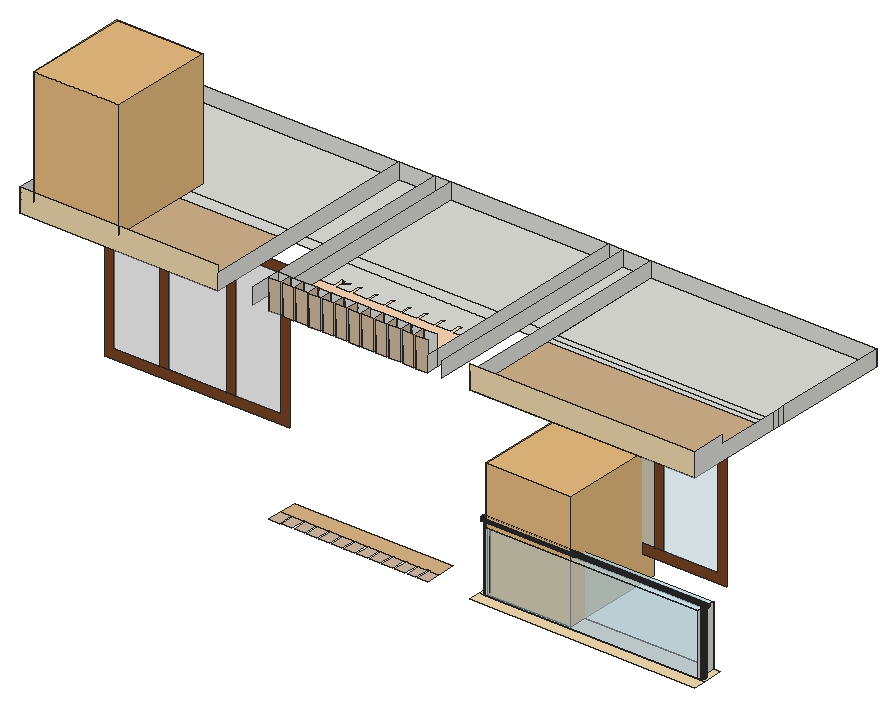
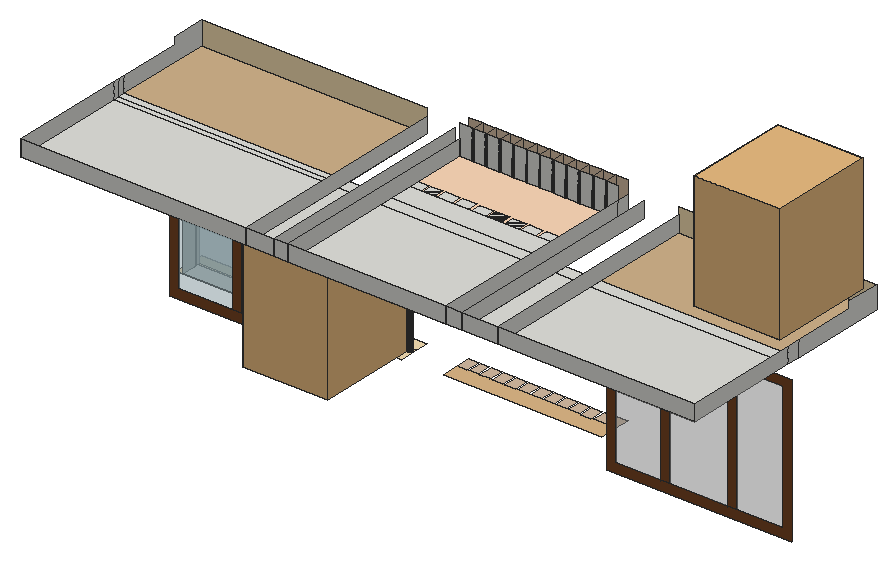
# SketchUp Ruby script. Lengths in inches.
U = 1.inch
M = Sketchup.active_model
def pt(a) = Geom::Point3d.new(a.map { |v| v * U })
def face(e, loops, mat)
  f = e.add_face(loops[0].map { |a| pt(a) })
  loops[1..].each { |l| e.add_face(l.map { |a| pt(a) }).erase! }
  f.material = f.back_material = mat if mat
  f
end
# faces: each face lists its corners as indices into pts; further lists are holes
def faces(e, pts, list, mat = nil) = list.each { |f| face(e, (f[0].is_a?(Array) ? f : [f]).map { |l| l.map { |i| pts[i] } }, mat) }
# xy, xz, yz: faces in a plane at the given z, y or x. An outline is a flat list of corners, or four numbers for a rectangle; further outlines are holes
def ring(l) = l.size == 4 ? [[l[0], l[1]], [l[2], l[1]], [l[2], l[3]], [l[0], l[3]]] : l.each_slice(2).to_a
def flat(e, list, mat, &to3) = list.each { |f| face(e, (f[0].is_a?(Array) ? f : [f]).map { |l| ring(l).map { |u, v| to3.(u, v) } }, mat) }
def xy(e, z, list, mat = nil) = flat(e, list, mat) { |x, y| [x, y, z] }
def xz(e, y, list, mat = nil) = flat(e, list, mat) { |x, z| [x, y, z] }
def yz(e, x, list, mat = nil) = flat(e, list, mat) { |y, z| [x, y, z] }
def lines(e, pts, list) = list.each { |a, b| e.add_line(pt(pts[a]), pt(pts[b])) }
# prism: a flat outline (further loops are holes) pulled along v
def prism(e, loops, v, mat = nil)
  f = face(e, loops, mat); d = Geom::Vector3d.new(v.map { |x| x * U })
  f.pushpull(f.normal.samedirection?(d) ? d.length : -d.length)
end
def box(e, o, s, mat = nil) = prism(e, [[o, [o[0] + s[0], o[1], o[2]], [o[0] + s[0], o[1] + s[1], o[2]], [o[0], o[1] + s[1], o[2]]]], [0, 0, s[2]], mat)
def at(x, y, z, deg = 0) = Geom::Transformation.translation(pt([x, y, z])) * Geom::Transformation.rotation(ORIGIN, Z_AXIS, deg.degrees)
def axes(o, x, y, z) = Geom::Transformation.new([*x, 0, *y, 0, *z, 0, *pt(o).to_a, 1])
def part(name) = M.definitions.add(name)
# library, detail: a bought-in or finely detailed component or shape, given as its bounding box
def library(name, o, s) = part(name).tap { |d| box(d.entities, o, s) }
def detail(e, o, s) = box(e.add_group.entities, o, s)
def put(e, d, t, mat = nil) = e.add_instance(d, t).tap { |i| i.material = mat if mat }
def group(e, t, mat = nil) = e.add_group.tap { |g| g.transformation = t; g.material = mat if mat }.entities
root = M.entities
M.materials.add("[0027_PeachPuff]").color = [255, 218, 185]
M.materials.add("[0034_Wheat]").color = [245, 222, 179]
M.materials.add("[0035_Tan]").color = [210, 180, 140]
M.materials.add("[0036_BurlyWood]1").color = [222, 184, 135]
M.materials.add("[Formica Laminate Dark]").color = [50, 53, 60]
M.materials.add("[Formica Laminate Light]").color = [213, 189, 164]
M.materials.add("[Translucent Glass Gray]").color = [191, 191, 191]
M.materials["[Translucent Glass Gray]"].alpha = 0.5
M.materials.add("[Translucent Glass Safety]").color = [204, 235, 244]
M.materials["[Translucent Glass Safety]"].alpha = 0.5
M.materials.add("[Wood Veneer 01]").color = [120, 70, 37]
c1 = library("chau cay",[-24.34,-109.24,0],[56.46,62.58,79.69])
xy(root,3893.0625,[[1416.35,332.76,2049.02,390.27],[1408.91,338.29,1408.19,338.33,1407.48,338.45,1406.79,338.64,1406.12,338.91,1405.48,339.24,1404.88,339.64,1404.33,340.1,1403.82,340.61,1403.375,341.18,1402.99,341.79,1402.67,342.43,1402.42,343.1,1402.24,343.8,1402.14,344.51,1402.11,345.23,1402.15,345.95,1402.27,346.66,1402.46,347.35,1402.73,348.02,1403.0625,348.66,1403.46,349.26,1403.92,349.8125,1404.43,350.32,1405,350.76,1405.6,351.15,1406.25,351.47,1406.92,351.72,1407.62,351.9,1408.33,352.01,1409.05,352.04,1409.77,351.99,1410.48,351.87,1411.17,351.68,1411.84,351.41,1412.47,351.07,1413.08,350.68,1413.63,350.22,1414.14,349.71,1414.58,349.14,1414.97,348.54,1415.29,347.89,1415.54,347.22,1415.72,346.52,1415.82,345.81,1415.85,345.09,1415.81,344.37,1415.6875,343.66,1415.5,342.97,1415.23,342.3,1414.9,341.66,1414.5,341.0625,1414.04,340.51,1413.53,340,1412.96,339.56,1412.36,339.17,1411.71,338.85,1411.04,338.6,1410.34,338.42,1409.63,338.32],[2056.54,338.29,2055.82,338.32,2055.11,338.4375,2054.42,338.62,2053.75,338.88,2053.1,339.21,2052.5,339.6,2051.94,340.05,2051.43,340.5625,2050.98,341.12,2050.59,341.72,2050.26,342.36,2050,343.04,2049.82,343.73,2049.7,344.44,2049.67,345.16,2049.7,345.88,2049.82,346.59,2050,347.29,2050.26,347.96,2050.59,348.6,2050.98,349.2,2051.43,349.76,2051.94,350.27,2052.5,350.72,2053.1,351.11,2053.75,351.44,2054.42,351.7,2055.11,351.89,2055.82,352,2056.54,352.04,2057.26,352,2057.97,351.89,2058.67,351.7,2059.34,351.44,2059.98,351.11,2060.58,350.72,2061.14,350.27,2061.65,349.76,2062.1,349.2,2062.5,348.6,2062.82,347.96,2063.08,347.29,2063.27,346.59,2063.38,345.88,2063.42,345.16,2063.38,344.44,2063.27,343.73,2063.08,343.04,2062.82,342.36,2062.5,341.72,2062.1,341.12,2061.65,340.5625,2061.14,340.05,2060.58,339.6,2059.98,339.21,2059.34,338.88,2058.67,338.62,2057.97,338.4375,2057.26,338.32]])
xy(root,3893.0625,[[1398.32,295.82,2069.85,332.76],[[1398.32,332.76,1416.35,390.27],[1408.91,338.29,1408.19,338.33,1407.48,338.45,1406.79,338.64,1406.12,338.91,1405.48,339.24,1404.88,339.64,1404.33,340.1,1403.82,340.61,1403.375,341.18,1402.99,341.79,1402.67,342.43,1402.42,343.1,1402.24,343.8,1402.14,344.51,1402.11,345.23,1402.15,345.95,1402.27,346.66,1402.46,347.35,1402.73,348.02,1403.0625,348.66,1403.46,349.26,1403.92,349.8125,1404.43,350.32,1405,350.76,1405.6,351.15,1406.25,351.47,1406.92,351.72,1407.62,351.9,1408.33,352.01,1409.05,352.04,1409.77,351.99,1410.48,351.87,1411.17,351.68,1411.84,351.41,1412.47,351.07,1413.08,350.68,1413.63,350.22,1414.14,349.71,1414.58,349.14,1414.97,348.54,1415.29,347.89,1415.54,347.22,1415.72,346.52,1415.82,345.81,1415.85,345.09,1415.81,344.37,1415.6875,343.66,1415.5,342.97,1415.23,342.3,1414.9,341.66,1414.5,341.0625,1414.04,340.51,1413.53,340,1412.96,339.56,1412.36,339.17,1411.71,338.85,1411.04,338.6,1410.34,338.42,1409.63,338.32]],[[2049.02,332.76,2069.85,390.27],[2056.54,338.29,2055.82,338.32,2055.11,338.4375,2054.42,338.62,2053.75,338.88,2053.1,339.21,2052.5,339.6,2051.94,340.05,2051.43,340.5625,2050.98,341.12,2050.59,341.72,2050.26,342.36,2050,343.04,2049.82,343.73,2049.7,344.44,2049.67,345.16,2049.7,345.88,2049.82,346.59,2050,347.29,2050.26,347.96,2050.59,348.6,2050.98,349.2,2051.43,349.76,2051.94,350.27,2052.5,350.72,2053.1,351.11,2053.75,351.44,2054.42,351.7,2055.11,351.89,2055.82,352,2056.54,352.04,2057.26,352,2057.97,351.89,2058.67,351.7,2059.34,351.44,2059.98,351.11,2060.58,350.72,2061.14,350.27,2061.65,349.76,2062.1,349.2,2062.5,348.6,2062.82,347.96,2063.08,347.29,2063.27,346.59,2063.38,345.88,2063.42,345.16,2063.38,344.44,2063.27,343.73,2063.08,343.04,2062.82,342.36,2062.5,341.72,2062.1,341.12,2061.65,340.5625,2061.14,340.05,2060.58,339.6,2059.98,339.21,2059.34,338.88,2058.67,338.62,2057.97,338.4375,2057.26,338.32]]],"[0034_Wheat]")
xy(root,3896.1875,[[800.41,338.63,1272.8,390.27]],"[0036_BurlyWood]1")
xy(root,3896.1875,[[800.41,295.82,831.22,338.63],[837.47,295.82,868.28,338.63],[875.6,295.82,906.41,338.63],[912.41,295.82,943.22,338.63],[949.16,295.82,979.97,338.63],
  [986.78,295.82,1017.6,338.63],[1024.35,295.82,1055.16,338.63],[1062.53,295.82,1093.35,338.63],[1100.28,295.82,1131.1,338.63],[1137.66,295.82,1168.47,338.63],
  [1175.22,295.82,1206.03,338.63],[1212.97,295.82,1238.19,338.63],[1243.78,295.82,1272.8,338.63]],"[Formica Laminate Light]")
xy(root,4072.9375,[[1416.35,332.76,2049.02,390.27]],"[Translucent Glass Safety]")
xy(root,4084.625,[[2056.54,338.29,2057.26,338.32,2057.97,338.4375,2058.67,338.62,2059.34,338.88,2059.98,339.21,2060.58,339.6,2061.14,340.05,2061.65,340.5625,2062.1,341.12,2062.5,341.72,2062.82,342.36,2063.08,343.04,2063.27,343.73,2063.38,344.44,2063.42,345.16,2063.38,345.88,2063.27,346.59,2063.08,347.29,2062.82,347.96,2062.5,348.6,2062.1,349.2,2061.65,349.76,2061.14,350.27,2060.58,350.72,2059.98,351.11,2059.34,351.44,2058.67,351.7,2057.97,351.89,2057.26,352,2056.54,352.04,2055.82,352,2055.11,351.89,2054.42,351.7,2053.75,351.44,2053.1,351.11,2052.5,350.72,2051.94,350.27,2051.43,349.76,2050.98,349.2,2050.59,348.6,2050.26,347.96,2050,347.29,2049.82,346.59,2049.7,345.88,2049.67,345.16,2049.7,344.44,2049.82,343.73,2050,343.04,2050.26,342.36,2050.59,341.72,2050.98,341.12,2051.43,340.5625,2051.94,340.05,2052.5,339.6,2053.1,339.21,2053.75,338.88,2054.42,338.62,2055.11,338.4375,2055.82,338.32]])
xy(root,4092.45,[[1408.91,338.29,1409.63,338.32,1410.34,338.42,1411.04,338.6,1411.71,338.85,1412.36,339.17,1412.96,339.56,1413.53,340,1414.04,340.51,1414.5,341.0625,1414.9,341.66,1415.23,342.3,1415.5,342.97,1415.6875,343.66,1415.81,344.37,1415.85,345.09,1415.82,345.81,1415.72,346.52,1415.54,347.22,1415.29,347.89,1414.97,348.54,1414.58,349.14,1414.42,349.34,1403.53,349.34,1403.46,349.26,1403.0625,348.66,1402.73,348.02,1402.46,347.35,1402.27,346.66,1402.15,345.95,1402.11,345.23,1402.14,344.51,1402.24,343.8,1402.42,343.1,1402.67,342.43,1402.99,341.79,1403.375,341.18,1403.82,340.61,1404.33,340.1,1404.88,339.64,1405.48,339.24,1406.12,338.91,1406.79,338.64,1407.48,338.45,1408.19,338.33],[1403.53,349.34,1414.42,349.34,1414.14,349.71,1413.63,350.22,1413.08,350.68,1412.47,351.07,1411.84,351.41,1411.17,351.68,1410.48,351.87,1409.77,351.99,1409.05,352.04,1408.33,352.01,1407.62,351.9,1406.92,351.72,1406.25,351.47,1405.6,351.15,1405,350.76,1404.43,350.32,1403.92,349.8125]])
xy(root,4453.25,[[800.41,483.92,800.41,584.29,1272.8,584.29,1272.8,483.92,1241.74,483.92,1241.74,514.17,1235.22,514.17,1235.22,483.92,1200.46,483.92,1200.46,514.17,1190.9375,514.17,1190.9375,483.92,1149.66,483.92,1149.66,514.17,1140.875,514.17,1140.875,483.92,1099.6,483.92,1099.6,514.17,1090.625,514.17,1090.625,483.92,1049.35,483.92,1049.35,514.17,1041.875,514.17,1041.875,483.92,1000.6,483.92,1000.6,514.17,991,514.17,991,483.92,949.72,483.92,949.72,514.17,942.25,514.17,942.25,483.92,900.97,483.92,900.97,514.17,891.6875,514.17,891.6875,483.92,850.41,483.92,850.41,514.17,841.6875,514.17,841.6875,483.92],[800.41,483.92,841.6875,514.17],[850.41,483.92,891.6875,514.17],[900.97,483.92,942.25,514.17],[949.72,483.92,991,514.17],
  [1000.6,483.92,1041.875,514.17],[1049.35,483.92,1090.625,514.17],[1099.6,483.92,1140.875,514.17],[1149.66,483.92,1190.9375,514.17],[1200.46,483.92,1235.22,514.17],
  [1241.74,483.92,1272.8,514.17],[800.41,514.17,1272.8,584.29],[58.44,584.29,646.67,623.89],[646.67,584.29,752.97,623.89],[752.97,584.29,800.41,623.89],
  [800.41,584.29,1272.8,623.89],[1272.8,584.29,1313.62,623.89],[1272.8,584.29,1313.62,623.89],[1313.62,584.29,1398.32,623.89],[1398.32,584.29,2069.85,604.09],
  [1398.32,604.09,2069.85,623.89],[58.44,623.89,646.67,971.67],[646.67,623.89,752.97,971.67],[752.97,623.89,800.41,971.67],[800.41,623.89,1272.8,971.67],
  [1272.8,623.89,1313.62,971.67],[1313.62,623.89,1398.32,971.67],[1398.32,623.89,2069.85,971.67]])
xy(root,4453.25,[[800.41,329.94,800.41,483.92,841.6875,483.92,841.6875,514.17,850.41,514.17,850.41,483.92,891.6875,483.92,891.6875,514.17,900.97,514.17,900.97,483.92,942.25,483.92,942.25,514.17,949.72,514.17,949.72,483.92,991,483.92,991,514.17,1000.6,514.17,1000.6,483.92,1041.875,483.92,1041.875,514.17,1049.35,514.17,1049.35,483.92,1090.625,483.92,1090.625,514.17,1099.6,514.17,1099.6,483.92,1140.875,483.92,1140.875,514.17,1149.66,514.17,1149.66,483.92,1190.9375,483.92,1190.9375,514.17,1200.46,514.17,1200.46,483.92,1235.22,483.92,1235.22,514.17,1241.74,514.17,1241.74,483.92,1272.8,483.92,1272.8,329.94]],"[0027_PeachPuff]")
xy(root,4453.25,[[58.44,295.82,646.67,584.29],[1398.32,295.82,2069.85,584.29]],"[0035_Tan]")
xy(root,4453.25,[[800.41,295.82,834.61,329.94],[840.03,295.82,874.24,329.94],[880.03,295.82,914.24,329.94],[919.91,295.82,954.11,329.94],[959.66,295.82,993.86,329.94],
  [998.72,295.82,1032.93,329.94],[1037.47,295.82,1071.68,329.94],[1076.91,295.82,1111.11,329.94],[1117.03,295.82,1151.24,329.94],[1157.28,295.82,1191.49,329.94],
  [1197.94,295.82,1232.15,329.94],[1238.6,295.82,1272.8,329.94]],"[Formica Laminate Light]")
xz(root,295.82,[[58.44,4453.25,646.67,4522.25],[1398.32,4453.25,2069.85,4522.25]],"[0034_Wheat]")
xz(root,295.82,[[800.41,4453.25,834.61,4541.3125],[840.03,4453.25,874.24,4541.3125],[880.03,4453.25,914.24,4541.3125],[919.91,4453.25,954.11,4541.3125],[959.66,4453.25,993.86,4541.3125],
  [998.72,4453.25,1032.93,4541.3125],[1037.47,4453.25,1071.68,4541.3125],[1076.91,4453.25,1111.11,4541.3125],[1117.03,4453.25,1151.24,4541.3125],[1157.28,4453.25,1191.49,4541.3125],
  [1197.94,4453.25,1232.15,4541.3125],[1238.6,4453.25,1272.8,4541.3125]],"[Formica Laminate Light]")
xz(root,329.94,[[800.41,4453.25,834.61,4541.3125],[840.03,4453.25,874.24,4541.3125],[880.03,4453.25,914.24,4541.3125],[919.91,4453.25,954.11,4541.3125],[959.66,4453.25,993.86,4541.3125],
  [998.72,4453.25,1032.93,4541.3125],[1037.47,4453.25,1071.68,4541.3125],[1076.91,4453.25,1111.11,4541.3125],[1117.03,4453.25,1151.24,4541.3125],[1157.28,4453.25,1191.49,4541.3125],
  [1197.94,4453.25,1232.15,4541.3125],[1238.6,4453.25,1272.8,4541.3125]])
xz(root,329.94,[[834.61,4453.25,840.03,4541.3125],[874.24,4453.25,880.03,4541.3125],[914.24,4453.25,919.91,4541.3125],[954.11,4453.25,959.66,4541.3125],[993.86,4453.25,998.72,4541.3125],
  [1032.93,4453.25,1037.47,4541.3125],[1071.68,4453.25,1076.91,4541.3125],[1111.11,4453.25,1117.03,4541.3125],[1151.24,4453.25,1157.28,4541.3125],[1191.49,4453.25,1197.94,4541.3125],
  [1232.15,4453.25,1238.6,4541.3125]],"[Formica Laminate Dark]")
xz(root,332.76,[[1416.35,3893.0625,2049.02,4072.9375]],"[Translucent Glass Safety]")
xz(root,390.27,[[1416.35,3893.0625,2049.02,4072.9375]],"[Translucent Glass Safety]")
xz(root,584.29,[[107.69,3981.23,243.82,4359.6875],[269.06,3981.23,444.26,4359.6875],[469.5,3981.23,603.34,4359.6875]],"[Translucent Glass Gray]")
xz(root,584.29,[[[80.45,3953.99,630.58,4386.93],[107.69,3981.23,603.34,4359.6875]],[243.82,3981.23,269.06,4359.6875],[444.26,3981.23,469.5,4359.6875]],"[Wood Veneer 01]")
xz(root,604.09,[[1550.67,4001.58,1704.3,4341.09],[1731.41,4001.58,1890.18,4341.09]],"[Translucent Glass Safety]")
xz(root,604.09,[[[1523.05,3973.96,1917.8,4368.71],[1550.67,4001.58,1890.18,4341.09]],[1704.3,4001.58,1731.41,4341.09]],"[Wood Veneer 01]")
xz(root,971.67,[[58.44,4453.25,646.67,4500.3125],[646.67,4453.25,752.97,4500.3125],[752.97,4453.25,800.41,4500.3125],[800.41,4453.25,1272.8,4500.3125],[1272.8,4453.25,1313.62,4500.3125],
  [1313.62,4453.25,1398.32,4500.3125],[1398.32,4453.25,2069.85,4500.3125]])
yz(root,58.44,[[295.82,4453.25,295.82,4522.25,397.09,4522.25,397.09,4500.3125,584.29,4500.3125,584.29,4453.25],[584.29,4453.25,623.89,4500.3125],[623.89,4453.25,971.67,4500.3125]])
yz(root,646.67,[[295.82,4453.25,971.67,4500.3125]])
yz(root,752.97,[[295.82,4453.25,971.67,4500.3125]])
yz(root,800.41,[[295.82,4453.25,329.94,4500.3125],[329.94,4453.25,971.67,4500.3125]])
yz(root,834.61,[[295.82,4453.25,329.94,4541.3125]],"[Formica Laminate Light]")
yz(root,840.03,[[295.82,4453.25,329.94,4500.3125]],"[Formica Laminate Light]")
yz(root,874.24,[[295.82,4453.25,329.94,4541.3125]],"[Formica Laminate Light]")
yz(root,880.03,[[295.82,4453.25,329.94,4500.3125]],"[Formica Laminate Light]")
yz(root,914.24,[[295.82,4453.25,329.94,4541.3125]],"[Formica Laminate Light]")
yz(root,919.91,[[295.82,4453.25,329.94,4500.3125]],"[Formica Laminate Light]")
yz(root,954.11,[[295.82,4453.25,329.94,4541.3125]],"[Formica Laminate Light]")
yz(root,959.66,[[295.82,4453.25,329.94,4500.3125]],"[Formica Laminate Light]")
yz(root,993.86,[[295.82,4453.25,329.94,4541.3125]],"[Formica Laminate Light]")
yz(root,998.72,[[295.82,4453.25,329.94,4500.3125]],"[Formica Laminate Light]")
yz(root,1032.93,[[295.82,4453.25,329.94,4541.3125]],"[Formica Laminate Light]")
yz(root,1037.47,[[295.82,4453.25,329.94,4500.3125]],"[Formica Laminate Light]")
yz(root,1071.68,[[295.82,4453.25,329.94,4541.3125]],"[Formica Laminate Light]")
yz(root,1076.91,[[295.82,4453.25,329.94,4500.3125]],"[Formica Laminate Light]")
yz(root,1111.11,[[295.82,4453.25,329.94,4541.3125]],"[Formica Laminate Light]")
yz(root,1117.03,[[295.82,4453.25,329.94,4500.3125]],"[Formica Laminate Light]")
yz(root,1151.24,[[295.82,4453.25,329.94,4541.3125]],"[Formica Laminate Light]")
yz(root,1157.28,[[295.82,4453.25,329.94,4500.3125]],"[Formica Laminate Light]")
yz(root,1191.49,[[295.82,4453.25,329.94,4541.3125]],"[Formica Laminate Light]")
yz(root,1197.94,[[295.82,4453.25,329.94,4500.3125]],"[Formica Laminate Light]")
yz(root,1232.15,[[295.82,4453.25,329.94,4541.3125]],"[Formica Laminate Light]")
yz(root,1238.6,[[295.82,4453.25,329.94,4500.3125]],"[Formica Laminate Light]")
yz(root,1272.8,[[295.82,4453.25,329.94,4500.3125],[329.94,4453.25,971.67,4500.3125]])
yz(root,1313.62,[[295.82,4453.25,971.67,4500.3125]])
yz(root,1398.32,[[295.82,4453.25,971.67,4500.3125]])
yz(root,1416.35,[[332.76,3893.0625,390.27,4072.9375]])
yz(root,2049.02,[[332.76,3893.0625,390.27,4072.9375]])
yz(root,2069.85,[[295.82,4453.25,584.29,4453.25,584.29,4500.3125,397.09,4500.3125,397.09,4522.25,295.82,4522.25],[584.29,4453.25,604.09,4500.3125],[604.09,4453.25,623.89,4500.3125],[623.89,4453.25,971.67,4500.3125]])
p = [[1407.48,338.45,3893.0625],[1408.19,338.33,3893.0625],[1408.19,338.33,4092.45],[1407.48,338.45,4092.45],[1408.91,338.29,3893.0625],[1408.91,338.29,4092.45],
  [1409.63,338.32,3893.0625],[1409.63,338.32,4092.45],[1410.34,338.42,3893.0625],[1410.34,338.42,4092.45],[2055.11,338.4375,3893.0625],[2055.82,338.32,3893.0625],
  [2055.82,338.32,4084.625],[2055.11,338.4375,4084.625],[2056.54,338.29,3893.0625],[2056.54,338.29,4084.625],[2057.26,338.32,3893.0625],[2057.26,338.32,4084.625],
  [2057.97,338.4375,3893.0625],[2057.97,338.4375,4084.625],[1411.04,338.6,3893.0625],[1411.04,338.6,4092.45],[2054.42,338.62,3893.0625],[2054.42,338.62,4084.625],
  [2058.67,338.62,3893.0625],[2058.67,338.62,4084.625],[1406.79,338.64,3893.0625],[1406.79,338.64,4092.45],[1406.12,338.91,3893.0625],[1406.12,338.91,4092.45],
  [1411.71,338.85,3893.0625],[1411.71,338.85,4092.45],[2053.75,338.88,3893.0625],[2053.75,338.88,4084.625],[2059.34,338.88,3893.0625],[2059.34,338.88,4084.625],
  [1405.48,339.24,3893.0625],[1405.48,339.24,4092.45],[1412.36,339.17,3893.0625],[1412.36,339.17,4092.45],[2053.1,339.21,3893.0625],[2053.1,339.21,4084.625],
  [2059.98,339.21,3893.0625],[2059.98,339.21,4084.625],[1404.88,339.64,3893.0625],[1404.88,339.64,4092.45],[1412.96,339.56,3893.0625],[1412.96,339.56,4092.45],
  [2052.5,339.6,3893.0625],[2052.5,339.6,4084.625],[2060.58,339.6,3893.0625],[2060.58,339.6,4084.625],[1404.33,340.1,3893.0625],[1404.33,340.1,4092.45],
  [1413.53,340,3893.0625],[1413.53,340,4092.45],[2051.94,340.05,3893.0625],[2051.94,340.05,4084.625],[2061.14,340.05,3893.0625],[2061.14,340.05,4084.625],
  [1414.04,340.51,3893.0625],[1414.04,340.51,4092.45],[1403.82,340.61,3893.0625],[1403.82,340.61,4092.45],[2051.43,340.5625,3893.0625],[2051.43,340.5625,4084.625],
  [2061.65,340.5625,3893.0625],[2061.65,340.5625,4084.625],[1414.5,341.0625,3893.0625],[1414.5,341.0625,4092.45],[1403.375,341.18,3893.0625],[1403.375,341.18,4092.45],
  [2050.98,341.12,3893.0625],[2050.98,341.12,4084.625],[2062.1,341.12,3893.0625],[2062.1,341.12,4084.625],[1414.9,341.66,3893.0625],[1414.9,341.66,4092.45],
  [2050.59,341.72,3893.0625],[2050.59,341.72,4084.625],[2062.5,341.72,3893.0625],[2062.5,341.72,4084.625],[1402.99,341.79,3893.0625],[1402.99,341.79,4092.45],
  [1415.23,342.3,3893.0625],[1415.23,342.3,4092.45],[2050.26,342.36,3893.0625],[2050.26,342.36,4084.625],[2062.82,342.36,3893.0625],[2062.82,342.36,4084.625],
  [1402.67,342.43,3893.0625],[1402.67,342.43,4092.45],[1415.5,342.97,3893.0625],[1415.5,342.97,4092.45],[1402.42,343.1,3893.0625],[1402.42,343.1,4092.45],
  [2050,343.04,3893.0625],[2050,343.04,4084.625],[2063.08,343.04,3893.0625],[2063.08,343.04,4084.625],[1415.6875,343.66,3893.0625],[1415.6875,343.66,4092.45],
  [2049.82,343.73,3893.0625],[2049.82,343.73,4084.625],[2063.27,343.73,3893.0625],[2063.27,343.73,4084.625],[1402.24,343.8,3893.0625],[1402.24,343.8,4092.45],
  [1415.81,344.37,3893.0625],[1415.81,344.37,4092.45],[2049.7,344.44,3893.0625],[2049.7,344.44,4084.625],[2063.38,344.44,3893.0625],[2063.38,344.44,4084.625],
  [1402.14,344.51,3893.0625],[1402.14,344.51,4092.45],[1415.85,345.09,3893.0625],[1415.85,345.09,4092.45],[2049.67,345.16,3893.0625],[2049.67,345.16,4084.625],
  [2063.42,345.16,3893.0625],[2063.42,345.16,4084.625],[1402.11,345.23,3893.0625],[1402.11,345.23,4092.45],[1415.82,345.81,3893.0625],[1415.82,345.81,4092.45],
  [1402.15,345.95,3893.0625],[1402.15,345.95,4092.45],[2049.7,345.88,3893.0625],[2049.7,345.88,4084.625],[2063.38,345.88,3893.0625],[2063.38,345.88,4084.625],
  [1415.72,346.52,3893.0625],[1415.72,346.52,4092.45],[2049.82,346.59,3893.0625],[2049.82,346.59,4084.625],[2063.27,346.59,3893.0625],[2063.27,346.59,4084.625],
  [1402.27,346.66,3893.0625],[1402.27,346.66,4092.45],[1415.54,347.22,3893.0625],[1415.54,347.22,4092.45],[2050,347.29,3893.0625],[2050,347.29,4084.625],
  [2063.08,347.29,3893.0625],[2063.08,347.29,4084.625],[1402.46,347.35,3893.0625],[1402.46,347.35,4092.45],[1415.29,347.89,3893.0625],[1415.29,347.89,4092.45],
  [2050.26,347.96,3893.0625],[2050.26,347.96,4084.625],[2062.82,347.96,3893.0625],[2062.82,347.96,4084.625],[1402.73,348.02,3893.0625],[1402.73,348.02,4092.45],
  [1414.97,348.54,3893.0625],[1414.97,348.54,4092.45],[1403.0625,348.66,3893.0625],[1403.0625,348.66,4092.45],[2050.59,348.6,3893.0625],[2050.59,348.6,4084.625],
  [2062.5,348.6,3893.0625],[2062.5,348.6,4084.625],[1414.58,349.14,3893.0625],[1414.58,349.14,4092.45],[2050.98,349.2,3893.0625],[2050.98,349.2,4084.625],
  [2062.1,349.2,3893.0625],[2062.1,349.2,4084.625],[1403.46,349.26,3893.0625],[1403.46,349.26,4092.45],[1414.14,349.71,3893.0625],[1414.14,349.71,4092.45],
  [1414.42,349.34,4092.45],[2051.43,349.76,3893.0625],[2051.43,349.76,4084.625],[2061.65,349.76,3893.0625],[2061.65,349.76,4084.625],[1403.92,349.8125,3893.0625],
  [1403.53,349.34,4092.45],[1403.92,349.8125,4092.45],[1413.63,350.22,3893.0625],[1413.63,350.22,4092.45],[1404.43,350.32,3893.0625],[1404.43,350.32,4092.45],
  [2051.94,350.27,3893.0625],[2051.94,350.27,4084.625],[2061.14,350.27,3893.0625],[2061.14,350.27,4084.625],[1413.08,350.68,3893.0625],[1413.08,350.68,4092.45],
  [1405,350.76,3893.0625],[1405,350.76,4092.45],[2052.5,350.72,3893.0625],[2052.5,350.72,4084.625],[2060.58,350.72,3893.0625],[2060.58,350.72,4084.625],
  [1412.47,351.07,3893.0625],[1412.47,351.07,4092.45],[2053.1,351.11,3893.0625],[2053.1,351.11,4084.625],[2059.98,351.11,3893.0625],[2059.98,351.11,4084.625],
  [1405.6,351.15,3893.0625],[1405.6,351.15,4092.45],[1411.84,351.41,3893.0625],[1411.84,351.41,4092.45],[2053.75,351.44,3893.0625],[2053.75,351.44,4084.625],
  [2059.34,351.44,3893.0625],[2059.34,351.44,4084.625],[1406.25,351.47,3893.0625],[1406.25,351.47,4092.45],[1411.17,351.68,3893.0625],[1411.17,351.68,4092.45],
  [2054.42,351.7,3893.0625],[2054.42,351.7,4084.625],[2058.67,351.7,3893.0625],[2058.67,351.7,4084.625],[1406.92,351.72,3893.0625],[1406.92,351.72,4092.45],
  [1407.62,351.9,3893.0625],[1407.62,351.9,4092.45],[1410.48,351.87,3893.0625],[1410.48,351.87,4092.45],[2055.11,351.89,3893.0625],[2055.11,351.89,4084.625],
  [2057.97,351.89,3893.0625],[2057.97,351.89,4084.625],[1408.33,352.01,3893.0625],[1408.33,352.01,4092.45],[1409.77,351.99,3893.0625],[1409.77,351.99,4092.45],
  [2055.82,352,3893.0625],[2055.82,352,4084.625],[2057.26,352,3893.0625],[2057.26,352,4084.625],[1409.05,352.04,3893.0625],[1409.05,352.04,4092.45],
  [2056.54,352.04,3893.0625],[2056.54,352.04,4084.625],[2069.85,343.39,4082.13],[2069.85,341.61,4082.37],[1398.32,341.61,4082.37],[1398.32,343.39,4082.13],
  [2069.85,345.17,4082.37],[1398.32,345.17,4082.37],[2069.85,339.95,4083.05],[1398.32,339.95,4083.05],[2069.85,346.83,4083.05],[1398.32,346.83,4083.05],
  [2069.85,338.53,4084.15],[1398.32,338.53,4084.15],[2069.85,348.25,4084.15],[1398.32,348.25,4084.15],[2069.85,337.4375,4085.57],[1398.32,337.4375,4085.57],
  [2069.85,349.34,4085.57],[1398.32,349.34,4085.57],[2069.85,336.75,4087.23],[1398.32,336.75,4087.23],[2069.85,350.03,4087.23],[1398.32,350.03,4087.23],
  [2069.85,336.52,4089.01],[1398.32,336.52,4089.01],[2069.85,350.27,4089.01],[1398.32,350.27,4089.01],[2069.85,336.75,4090.79],[1398.32,336.75,4090.79],
  [2069.85,350.03,4090.79],[1398.32,350.03,4090.79],[2069.85,337.4375,4092.45],[1398.32,337.4375,4092.45],[2069.85,349.34,4092.45],[1398.32,349.34,4092.45],
  [2069.85,338.53,4093.87],[1398.32,338.53,4093.87],[2069.85,348.25,4093.87],[1398.32,348.25,4093.87],[2069.85,339.95,4094.96],[1398.32,339.95,4094.96],
  [2069.85,346.83,4094.96],[1398.32,346.83,4094.96],[2069.85,341.61,4095.65],[1398.32,341.61,4095.65],[2069.85,345.17,4095.65],[1398.32,345.17,4095.65],
  [2069.85,343.39,4095.88],[1398.32,343.39,4095.88]]
faces(root,p,[[0,1,2,3],[1,4,5,2],[4,6,7,5],[6,8,9,7],[10,11,12,13],[11,14,15,12],[14,16,17,15],[16,18,19,17],
  [8,20,21,9],[22,10,13,23],[18,24,25,19],[26,0,3,27],[28,26,27,29],[20,30,31,21],[32,22,23,33],[24,34,35,25],
  [36,28,29,37],[30,38,39,31],[40,32,33,41],[34,42,43,35],[44,36,37,45],[38,46,47,39],[48,40,41,49],[42,50,51,43],
  [52,44,45,53],[46,54,55,47],[56,48,49,57],[50,58,59,51],[54,60,61,55],[62,52,53,63],[64,56,57,65],[58,66,67,59],
  [60,68,69,61],[70,62,63,71],[72,64,65,73],[66,74,75,67],[68,76,77,69],[78,72,73,79],[74,80,81,75],[82,70,71,83],
  [76,84,85,77],[86,78,79,87],[80,88,89,81],[90,82,83,91],[84,92,93,85],[94,90,91,95],[96,86,87,97],[88,98,99,89],
  [92,100,101,93],[102,96,97,103],[98,104,105,99],[106,94,95,107],[100,108,109,101],[110,102,103,111],[104,112,113,105],[114,106,107,115],
  [108,116,117,109],[118,110,111,119],[112,120,121,113],[122,114,115,123],[116,124,125,117],[126,122,123,127],[128,118,119,129],[120,130,131,121],
  [124,132,133,125],[134,128,129,135],[130,136,137,131],[138,126,127,139],[132,140,141,133],[142,134,135,143],[136,144,145,137],[146,138,139,147],
  [140,148,149,141],[150,142,143,151],[144,152,153,145],[154,146,147,155],[148,156,157,149],[158,154,155,159],[160,150,151,161],[152,162,163,153],
  [156,164,165,157],[166,160,161,167],[162,168,169,163],[170,158,159,171],[164,172,173,174,165],[175,166,167,176],[168,177,178,169],[179,170,171,180,181],
  [172,182,183,173],[184,179,181,185],[186,175,176,187],[177,188,189,178],[182,190,191,183],[192,184,185,193],[194,186,187,195],[188,196,197,189],
  [190,198,199,191],[200,194,195,201],[196,202,203,197],[204,192,193,205],[198,206,207,199],[208,200,201,209],[202,210,211,203],[212,204,205,213],
  [206,214,215,207],[216,208,209,217],[210,218,219,211],[220,212,213,221],[222,220,221,223],[214,224,225,215],[226,216,217,227],[218,228,229,219],
  [230,222,223,231],[224,232,233,225],[234,226,227,235],[228,236,237,229],[238,230,231,239],[232,238,239,233],[240,234,235,241],[236,240,241,237],
  [242,243,244,245],[246,242,245,247],[243,248,249,244],[250,246,247,251],[248,252,253,249],[254,250,251,255],[252,256,257,253],[258,254,255,259],
  [256,260,261,257],[262,258,259,263],[260,264,265,261],[266,262,263,267],[264,268,269,265],[270,266,267,271],[268,272,273,269],[274,270,271,275,180,174],
  [272,276,277,273],[278,274,174,180,275,279],[276,280,281,277],[282,278,279,283],[280,284,285,281],[286,282,283,287],[284,288,289,285],[288,286,287,289]],"[Formica Laminate Dark]")
put(root,c1,axes([1520.56,106.94,3893.0625],[4.5,0,0],[0,-4.9651,0],[0,0,4.37432]))
put(root,c1,axes([208.02,64.16,4497.5],[4.5,0,0],[0,-4.9651,0],[0,0,4.37432]))
